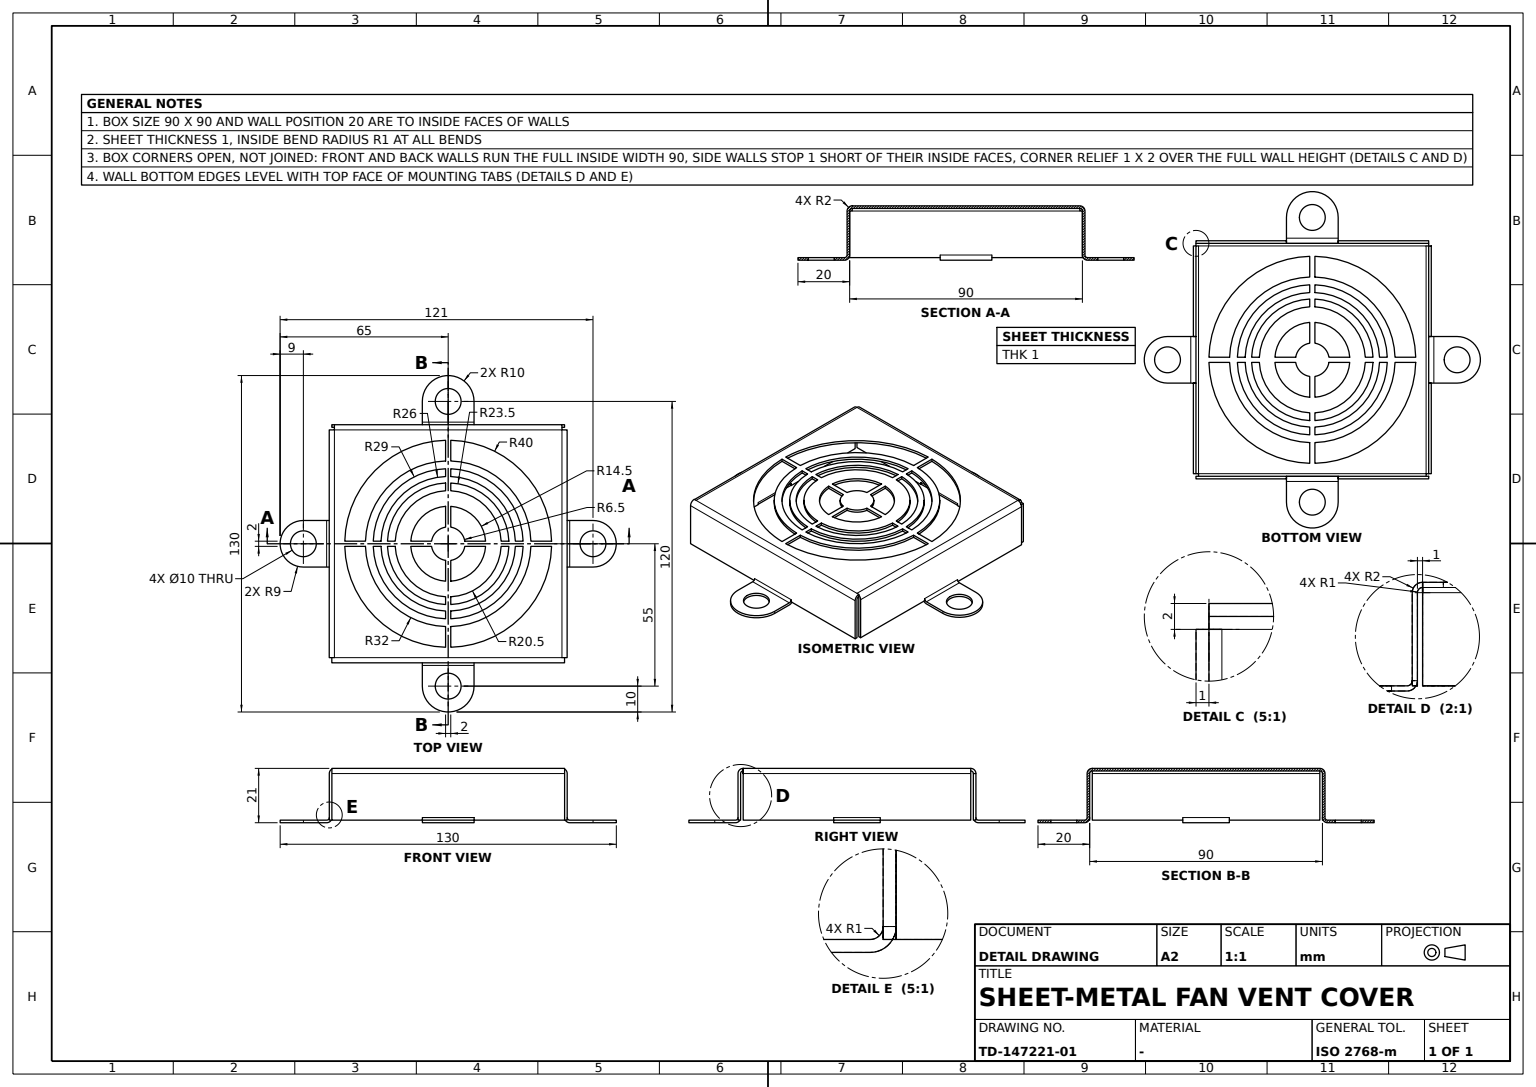
solid
v1 (14.465476,-1,0)
v2 (14.465476,-1,1)
e1 v1 v2 LINE
v3 (6.422616,-1,1)
e2 v2 v3 LINE
v4 (6.422616,-1,0)
e3 v4 v3 LINE
e4 v1 v4 LINE
face PLANE(AX(P(-10.444046,-1,1),D(0,1,0),D(1,0,0))) rev [e1 e2 -e3 -e4]
v5 (1,25.982753,1)
v6 (25.982753,1,1)
e5 v5 v6 CIRCLE(AX(P(0,0,1),D(0,0,1),D(1,0,0)),26.00199) rev
v7 (25.982753,1,0)
e6 v7 v6 LINE
v8 (1,25.982753,0)
e7 v8 v7 CIRCLE(AX(P(0,0,0),D(0,0,1),D(1,0,0)),26.00199) rev
e8 v8 v5 LINE
face CYL(AX(P(0,0,1),D(0,0,1),D(0,1,0)),26.00199) [e5 -e6 -e7 e8]
v9 (-56,9,-20)
v10 (-55.999997,9,-19)
e9 v9 v10 LINE
v11 (-47,9,-19)
e10 v10 v11 LINE
v12 (-46,9,-18)
e11 v11 v12 CIRCLE(AX(P(-47,9,-18),D(0,-1,0),D(0,0,-1)),1)
v13 (-45,9,-18)
e12 v13 v12 LINE
v14 (-47,9,-20)
e13 v14 v13 CIRCLE(AX(P(-47,9,-18),D(0,-1,0),D(0,0,-1)),2)
e14 v9 v14 LINE
face PLANE(AX(P(56,9,-20),D(0,-1,0),D(1,0,0))) rev [e9 e10 e11 -e12 -e13 -e14]
v15 (-61,0,-20)
e15 v15 v15 CIRCLE(AX(P(-56,0,-20),D(0,0,-1),D(-1,0,0)),5) rev
v16 (-61,0,-19)
e16 v16 v16 CIRCLE(AX(P(-56,0,-19),D(0,0,-1),D(-1,0,0)),5) rev
face CYL(AX(P(-56,0,-19),D(0,0,-1),D(0,1,0)),5) rev [-e15] [e16]
v17 (-1,-14.465476,0)
v18 (-14.465476,-1,0)
e17 v17 v18 CIRCLE(AX(P(0,0,0),D(0,0,1),D(1,0,0)),14.5) rev
v19 (-14.465476,-1,1)
e18 v18 v19 LINE
v20 (-1,-14.465476,1)
e19 v20 v19 CIRCLE(AX(P(0,0,1),D(0,0,1),D(1,0,0)),14.5) rev
e20 v17 v20 LINE
face CYL(AX(P(0,0,1),D(0,0,1),D(0,1,0)),14.5) rev [e17 e18 -e19 -e20]
v21 (-56,-9,-20)
e21 v21 v9 CIRCLE(AX(P(-56,0,-20),D(0,0,-1),D(-1,0,0)),9)
v22 (-56,-9,-19)
e22 v21 v22 LINE
e23 v22 v10 CIRCLE(AX(P(-56,0,-19),D(0,0,-1),D(-1,0,0)),9)
face CYL(AX(P(-56,0,-19),D(0,0,-1),D(0,1,0)),9) [-e9 -e21 e22 e23]
v23 (10,45,-18)
v24 (10,45,-19)
e24 v23 v24 LINE
v25 (10,46,-18)
e25 v23 v25 LINE
v26 (10,46,-19)
e26 v25 v26 LINE
e27 v24 v26 LINE
face PLANE(AX(P(10,-45,-18),D(-1,0,0),D(0,-0.382683432,-0.923879533))) [-e24 e25 e26 -e27]
v27 (-31.984371,-1,0)
v28 (-31.984371,-1,1)
e28 v27 v28 LINE
v29 (-1,-31.984371,0)
e29 v27 v29 CIRCLE(AX(P(0,0,0),D(0,0,1),D(1,0,0)),32)
v30 (-1,-31.984371,1)
e30 v29 v30 LINE
e31 v28 v30 CIRCLE(AX(P(0,0,1),D(0,0,1),D(1,0,0)),32)
face CYL(AX(P(0,0,1),D(0,0,1),D(0,1,0)),32) [-e28 e29 e30 -e31]
v31 (1,-14.465476,0)
e32 v1 v31 CIRCLE(AX(P(0,0,0),D(0,0,1),D(1,0,0)),14.5) rev
v32 (1,-14.465476,1)
e33 v31 v32 LINE
e34 v2 v32 CIRCLE(AX(P(0,0,1),D(0,0,1),D(1,0,0)),14.5) rev
face CYL(AX(P(0,0,1),D(0,0,1),D(0,1,0)),14.5) rev [e32 e33 -e34 -e1]
v33 (-45,46,-19)
v34 (-45,46,-1)
e35 v33 v34 LINE
v35 (-45,45,-19)
e36 v35 v33 LINE
v36 (-45,45,-1)
e37 v35 v36 LINE
e38 v36 v34 LINE
face PLANE(AX(P(-45,46,-10),D(-1,0,0),D(0,1,0))) [-e35 -e36 e37 e38]
v37 (1,14.465476,1)
v38 (14.465476,1,1)
e39 v37 v38 CIRCLE(AX(P(0,0,1),D(0,0,1),D(1,0,0)),14.5) rev
v39 (1,14.465476,0)
e40 v39 v37 LINE
v40 (14.465476,1,0)
e41 v39 v40 CIRCLE(AX(P(0,0,0),D(0,0,1),D(1,0,0)),14.5) rev
e42 v40 v38 LINE
face CYL(AX(P(0,0,1),D(0,0,1),D(0,1,0)),14.5) rev [-e39 -e40 e41 e42]
v41 (6.422616,1,0)
e43 v41 v40 LINE
v42 (6.422616,1,1)
e44 v41 v42 LINE
e45 v42 v38 LINE
face PLANE(AX(P(-10.444046,1,1),D(0,1,0),D(1,0,0))) [-e42 -e43 e44 e45]
v43 (-46,44,-19)
v44 (-46,9,-19)
e46 v43 v44 LINE
v45 (-45,44,-19)
e47 v43 v45 LINE
v46 (-45,9,-19)
e48 v45 v46 LINE
e49 v46 v44 LINE
face PLANE(AX(P(46,0,-19),D(0,0,-1),D(0,1,0))) [-e46 e47 e48 e49]
v47 (-1,14.465476,0)
v48 (-1,14.465476,1)
e50 v47 v48 LINE
v49 (-14.465476,1,1)
e51 v48 v49 CIRCLE(AX(P(0,0,1),D(0,0,1),D(1,0,0)),14.5)
v50 (-14.465476,1,0)
e52 v50 v49 LINE
e53 v47 v50 CIRCLE(AX(P(0,0,0),D(0,0,1),D(1,0,0)),14.5)
face CYL(AX(P(0,0,1),D(0,0,1),D(0,1,0)),14.5) rev [e50 e51 -e52 -e53]
v51 (45,45,-1)
v52 (45,46,-1)
e54 v51 v52 LINE
v53 (45,45,-19)
e55 v53 v51 LINE
v54 (45,46,-19)
e56 v53 v54 LINE
e57 v54 v52 LINE
face PLANE(AX(P(45,0,1),D(-1,0,0),D(0,1,0))) rev [-e54 -e55 e56 e57]
v55 (-45,-9,-18)
v56 (-46,-9,-18)
e58 v55 v56 LINE
v57 (-45,-9,-19)
e59 v55 v57 LINE
v58 (-46,-9,-19)
e60 v57 v58 LINE
e61 v56 v58 LINE
face PLANE(AX(P(56,-9,-20),D(0,-1,0),D(1,0,0))) rev [-e58 e59 e60 -e61]
e62 v12 v44 LINE
e63 v56 v12 LINE
v59 (-46,-44,-19)
e64 v58 v59 LINE
v60 (-46,-44,-1)
e65 v59 v60 LINE
v61 (-46,44,-1)
e66 v60 v61 LINE
e67 v61 v43 LINE
face PLANE(AX(P(-46,0,1),D(-1,0,0),D(0,1,0))) [e46 -e62 -e63 e61 e64 e65 e66 e67]
v62 (-1,25.982753,0)
v63 (-1,25.982753,1)
e68 v62 v63 LINE
v64 (-25.982753,1,0)
e69 v62 v64 CIRCLE(AX(P(0,0,0),D(0,0,1),D(1,0,0)),26.00199)
v65 (-25.982753,1,1)
e70 v64 v65 LINE
e71 v63 v65 CIRCLE(AX(P(0,0,1),D(0,0,1),D(1,0,0)),26.00199)
face CYL(AX(P(0,0,1),D(0,0,1),D(0,1,0)),26.00199) [-e68 e69 e70 -e71]
v66 (10,54.999996,-19)
v67 (10,47,-19)
e72 v66 v67 LINE
v68 (-10,55,-19)
e73 v68 v66 CIRCLE(AX(P(0,55,-19),D(0,0,-1),D(-1,0,0)),10)
v69 (-10,47,-19)
e74 v68 v69 LINE
e75 v67 v69 LINE
v70 (-5,55,-19)
e76 v70 v70 CIRCLE(AX(P(0,55,-19),D(0,0,-1),D(-1,0,0)),5) rev
face PLANE(AX(P(46,0,-19),D(0,0,-1),D(0,1,0))) rev [-e72 -e73 e74 -e75] [-e76]
e77 v54 v26 LINE
v71 (-10,46,-18)
e78 v25 v71 LINE
v72 (-10,46,-19)
e79 v71 v72 LINE
e80 v72 v33 LINE
v73 (-44,46,-1)
e81 v34 v73 LINE
v74 (44,46,-1)
e82 v74 v73 LINE
e83 v74 v52 LINE
face PLANE(AX(P(0,46,1),D(0,-1,0),D(-1,0,0))) rev [e77 -e26 e78 e79 e80 e35 e81 -e82 e83 -e57]
v75 (-6.422616,-1,0)
v76 (-6.422616,-1,1)
e84 v75 v76 LINE
v77 (-1,-6.422616,0)
e85 v77 v75 CIRCLE(AX(P(0,0,0),D(0,0,1),D(1,0,0)),6.5) rev
v78 (-1,-6.422616,1)
e86 v77 v78 LINE
e87 v78 v76 CIRCLE(AX(P(0,0,1),D(0,0,1),D(1,0,0)),6.5) rev
face CYL(AX(P(0,0,1),D(0,0,1),D(0,1,0)),6.5) [-e84 -e85 e86 e87]
v79 (1,28.982753,0)
v80 (1,28.982753,1)
e88 v79 v80 LINE
e89 v5 v80 LINE
e90 v8 v79 LINE
face PLANE(AX(P(1,-10.444046,1),D(1,0,0),D(0,1,0))) [e88 -e89 -e8 e90]
v81 (39.987498,-1,0)
v82 (39.987498,-1,1)
e91 v81 v82 LINE
v83 (31.984371,-1,1)
e92 v83 v82 LINE
v84 (31.984371,-1,0)
e93 v84 v83 LINE
e94 v84 v81 LINE
face PLANE(AX(P(-10.444046,-1,1),D(0,1,0),D(1,0,0))) rev [e91 -e92 -e93 e94]
v85 (47,-9,-20)
v86 (47,9,-20)
e95 v85 v86 LINE
v87 (56,9,-20)
e96 v87 v86 LINE
v88 (56,-9,-20)
e97 v87 v88 CIRCLE(AX(P(56,0,-20),D(0,0,-1),D(-1,0,0)),9)
e98 v85 v88 LINE
v89 (51,0,-20)
e99 v89 v89 CIRCLE(AX(P(56,0,-20),D(0,0,-1),D(-1,0,0)),5)
face PLANE(AX(P(46,0,-20),D(0,0,-1),D(0,1,0))) [e95 -e96 e97 -e98] [-e99]
v90 (47,-9,-19)
v91 (56,-9,-19)
e100 v90 v91 LINE
v92 (46,-9,-18)
e101 v92 v90 CIRCLE(AX(P(47,-9,-18),D(0,-1,0),D(0,0,-1)),1)
v93 (45,-9,-18)
e102 v93 v92 LINE
e103 v93 v85 CIRCLE(AX(P(47,-9,-18),D(0,-1,0),D(0,0,-1)),2)
e104 v88 v91 LINE
face PLANE(AX(P(56,-9,-20),D(0,-1,0),D(1,0,0))) [-e100 -e101 -e102 e103 e98 e104]
v94 (46,-44,-1)
v95 (44,-44,1)
e105 v94 v95 CIRCLE(AX(P(44,-44,-1),D(0,1,0),D(0,0,1)),2) rev
v96 (46,44,-1)
e106 v94 v96 LINE
v97 (44,44,1)
e107 v96 v97 CIRCLE(AX(P(44,44,-1),D(0,1,0),D(0,0,1)),2) rev
e108 v95 v97 LINE
face CYL(AX(P(44,-44,-1),D(0,1,0),D(0,0,1)),2) [-e105 e106 e107 -e108]
v98 (10,-45,-18)
v99 (10,-45,-19)
e109 v98 v99 LINE
v100 (10,-46,-19)
e110 v99 v100 LINE
v101 (10,-46,-18)
e111 v101 v100 LINE
e112 v98 v101 LINE
face PLANE(AX(P(10,-45,-18),D(-1,0,0),D(0,-0.382683432,-0.923879533))) [e109 e110 -e111 -e112]
v102 (-44,44,0)
v103 (-45,44,-1)
e113 v102 v103 CIRCLE(AX(P(-44,44,-1),D(0,1,0),D(0,0,1)),1) rev
v104 (-44,-44,0)
e114 v104 v102 LINE
v105 (-45,-44,-1)
e115 v104 v105 CIRCLE(AX(P(-44,-44,-1),D(0,1,0),D(0,0,1)),1) rev
e116 v105 v103 LINE
face CYL(AX(P(-44,44,-1),D(0,-1,0),D(0,0,1)),1) rev [-e113 -e114 e115 e116]
v106 (1,-39.987498,0)
v107 (1,-39.987498,1)
e117 v106 v107 LINE
v108 (1,-31.984371,0)
e118 v108 v106 LINE
v109 (1,-31.984371,1)
e119 v108 v109 LINE
e120 v109 v107 LINE
face PLANE(AX(P(1,-10.444046,1),D(1,0,0),D(0,1,0))) [-e117 -e118 e119 e120]
v110 (-28.982753,-1,0)
v111 (-28.982753,-1,1)
e121 v110 v111 LINE
v112 (-1,-28.982753,1)
e122 v112 v111 CIRCLE(AX(P(0,0,1),D(0,0,1),D(1,0,0)),29) rev
v113 (-1,-28.982753,0)
e123 v113 v112 LINE
e124 v113 v110 CIRCLE(AX(P(0,0,0),D(0,0,1),D(1,0,0)),29) rev
face CYL(AX(P(0,0,1),D(0,0,1),D(0,1,0)),29) rev [e121 -e122 -e123 e124]
v114 (45,44,-1)
v115 (44,44,0)
e125 v114 v115 CIRCLE(AX(P(44,44,-1),D(0,1,0),D(0,0,1)),1) rev
v116 (45,-44,-1)
e126 v116 v114 LINE
v117 (44,-44,0)
e127 v116 v117 CIRCLE(AX(P(44,-44,-1),D(0,1,0),D(0,0,1)),1) rev
e128 v117 v115 LINE
face CYL(AX(P(44,-44,-1),D(0,1,0),D(0,0,1)),1) rev [-e125 -e126 e127 e128]
v118 (-31.984371,1,0)
v119 (-39.987498,1,0)
e129 v118 v119 LINE
v120 (-39.987498,1,1)
e130 v119 v120 LINE
v121 (-31.984371,1,1)
e131 v121 v120 LINE
e132 v118 v121 LINE
face PLANE(AX(P(-10.444046,1,1),D(0,1,0),D(1,0,0))) [e129 e130 -e131 -e132]
v122 (39.987498,1,0)
v123 (31.984371,1,0)
e133 v122 v123 LINE
v124 (31.984371,1,1)
e134 v123 v124 LINE
v125 (39.987498,1,1)
e135 v125 v124 LINE
e136 v122 v125 LINE
face PLANE(AX(P(-10.444046,1,1),D(0,1,0),D(1,0,0))) [e133 e134 -e135 -e136]
v126 (25.982753,-1,0)
v127 (25.982753,-1,1)
e137 v126 v127 LINE
v128 (28.982753,-1,0)
e138 v126 v128 LINE
v129 (28.982753,-1,1)
e139 v128 v129 LINE
e140 v127 v129 LINE
face PLANE(AX(P(-10.444046,-1,1),D(0,1,0),D(1,0,0))) rev [-e137 e138 e139 -e140]
v130 (10,47,-20)
e141 v23 v130 CIRCLE(AX(P(10,47,-18),D(-1,0,0),D(0,0,1)),2) rev
v131 (-10,45,-18)
e142 v23 v131 LINE
v132 (-10,47,-20)
e143 v131 v132 CIRCLE(AX(P(-10,47,-18),D(-1,0,0),D(0,0,1)),2) rev
e144 v130 v132 LINE
face CYL(AX(P(-10,47,-18),D(1,0,0),D(0,-1,0)),2) [-e141 e142 e143 -e144]
v133 (1,-6.422616,0)
e145 v31 v133 LINE
v134 (1,-6.422616,1)
e146 v133 v134 LINE
e147 v32 v134 LINE
face PLANE(AX(P(1,-10.444046,1),D(1,0,0),D(0,1,0))) [-e33 e145 e146 -e147]
v135 (1,-25.982753,0)
e148 v135 v126 CIRCLE(AX(P(0,0,0),D(0,0,1),D(1,0,0)),26.00199)
v136 (1,-25.982753,1)
e149 v136 v127 CIRCLE(AX(P(0,0,1),D(0,0,1),D(1,0,0)),26.00199)
e150 v135 v136 LINE
face CYL(AX(P(0,0,1),D(0,0,1),D(0,1,0)),26.00199) [e148 e137 -e149 -e150]
v137 (45,-45,-1)
v138 (-45,-45,-1)
e151 v137 v138 LINE
v139 (-45,-44,0)
e152 v139 v138 CIRCLE(AX(P(-45,-44,-1),D(-1,0,0),D(0,0,1)),1) rev
e153 v139 v104 LINE
e154 v117 v104 LINE
v140 (45,-44,0)
e155 v140 v117 LINE
e156 v140 v137 CIRCLE(AX(P(45,-44,-1),D(-1,0,0),D(0,0,1)),1) rev
face CYL(AX(P(-45,-44,-1),D(1,0,0),D(0,0,1)),1) rev [e151 -e152 e153 -e154 -e155 e156]
v141 (46,-9,-19)
e157 v92 v141 LINE
v142 (45,-9,-19)
e158 v142 v141 LINE
e159 v93 v142 LINE
face PLANE(AX(P(56,-9,-20),D(0,-1,0),D(1,0,0))) rev [e157 -e158 -e159 e102]
v143 (-28.982753,1,1)
e160 v65 v143 LINE
v144 (-28.982753,1,0)
e161 v64 v144 LINE
e162 v144 v143 LINE
face PLANE(AX(P(-10.444046,1,1),D(0,1,0),D(1,0,0))) [-e160 -e70 e161 e162]
v145 (-44,44,1)
e163 v102 v145 LINE
e164 v145 v73 CIRCLE(AX(P(-44,44,-1),D(-1,0,0),D(0,0,1)),2)
v146 (-44,45,-1)
e165 v146 v73 LINE
e166 v102 v146 CIRCLE(AX(P(-44,44,-1),D(-1,0,0),D(0,0,1)),1)
face PLANE(AX(P(-44,44,0),D(-1,0,0),D(0,0.923879533,-0.382683432))) [e163 e164 -e165 -e166]
v147 (44,45,-1)
e167 v147 v51 LINE
e168 v147 v146 LINE
e169 v36 v146 LINE
v148 (-10,45,-19)
e170 v35 v148 LINE
e171 v131 v148 LINE
e172 v24 v53 LINE
face PLANE(AX(P(0,45,1),D(0,-1,0),D(-1,0,0))) [-e167 e168 -e169 -e37 e170 -e171 -e142 e24 e172 e55]
v149 (45,-44,1)
e173 v149 v95 LINE
e174 v140 v149 LINE
e175 v117 v95 LINE
face PLANE(AX(P(46,-44,-10),D(0,1,0),D(1,0,0))) [-e173 -e174 e155 e175]
v150 (-5,-55,-20)
e176 v150 v150 CIRCLE(AX(P(0,-55,-20),D(0,0,-1),D(-1,0,0)),5) rev
v151 (-5,-55,-19)
e177 v151 v151 CIRCLE(AX(P(0,-55,-19),D(0,0,-1),D(-1,0,0)),5) rev
face CYL(AX(P(0,-55,-19),D(0,0,-1),D(-1,0,0)),5) rev [-e176] [e177]
v152 (45,44,-19)
e178 v152 v114 LINE
v153 (45,9,-19)
e179 v152 v153 LINE
v154 (45,9,-18)
e180 v154 v153 LINE
e181 v93 v154 LINE
v155 (45,-44,-19)
e182 v142 v155 LINE
e183 v116 v155 LINE
face PLANE(AX(P(45,0,1),D(-1,0,0),D(0,1,0))) [-e178 e179 -e180 -e181 e159 e182 -e183 e126]
v156 (23.478714,1,0)
v157 (1,23.478714,0)
e184 v156 v157 CIRCLE(AX(P(0,0,0),D(0,0,1),D(1,0,0)),23.5)
v158 (23.478714,1,1)
e185 v156 v158 LINE
v159 (1,23.478714,1)
e186 v158 v159 CIRCLE(AX(P(0,0,1),D(0,0,1),D(1,0,0)),23.5)
e187 v157 v159 LINE
face CYL(AX(P(0,0,1),D(0,0,1),D(0,1,0)),23.5) rev [-e184 e185 e186 -e187]
v160 (10,-47,-20)
e188 v160 v98 CIRCLE(AX(P(10,-47,-18),D(-1,0,0),D(0,0,1)),2) rev
v161 (10,-47,-19)
e189 v161 v101 CIRCLE(AX(P(10,-47,-18),D(-1,0,0),D(0,0,1)),1) rev
v162 (10,-55,-19)
e190 v162 v161 LINE
v163 (10,-54.999996,-20)
e191 v163 v162 LINE
e192 v163 v160 LINE
face PLANE(AX(P(10,-45,-18),D(-1,0,0),D(0,-0.382683432,-0.923879533))) rev [e188 e112 -e189 -e190 -e191 e192]
e193 v109 v83 CIRCLE(AX(P(0,0,1),D(0,0,1),D(1,0,0)),32)
e194 v108 v84 CIRCLE(AX(P(0,0,0),D(0,0,1),D(1,0,0)),32)
face CYL(AX(P(0,0,1),D(0,0,1),D(0,1,0)),32) [-e193 -e119 e194 e93]
v164 (-10,-55,-19)
v165 (-10,-47,-19)
e195 v164 v165 LINE
e196 v162 v164 CIRCLE(AX(P(0,-55,-19),D(0,0,-1),D(-1,0,0)),10)
e197 v161 v165 LINE
face PLANE(AX(P(46,0,-19),D(0,0,-1),D(0,1,0))) rev [-e195 -e196 e190 e197] [-e177]
v166 (-45,-44,1)
v167 (-44,-44,1)
e198 v166 v167 LINE
e199 v104 v167 LINE
e200 v139 v166 LINE
face PLANE(AX(P(46,-44,-10),D(0,1,0),D(1,0,0))) [e198 -e199 -e153 e200]
v168 (-10,-55,-20)
e201 v163 v168 CIRCLE(AX(P(0,-55,-20),D(0,0,-1),D(-1,0,0)),10)
v169 (-10,-47,-20)
e202 v168 v169 LINE
e203 v160 v169 LINE
face PLANE(AX(P(46,0,-20),D(0,0,-1),D(0,1,0))) [e201 e202 -e203 -e192] [e176]
e204 v131 v71 LINE
e205 v148 v72 LINE
face PLANE(AX(P(-10,-45,-18),D(-1,0,0),D(0,-0.382683432,-0.923879533))) rev [-e204 e171 e205 -e79]
v170 (20.478714,1,1)
e206 v158 v170 LINE
v171 (20.478714,1,0)
e207 v156 v171 LINE
e208 v171 v170 LINE
face PLANE(AX(P(-10.444046,1,1),D(0,1,0),D(1,0,0))) [-e206 -e185 e207 e208]
v172 (46,9,-19)
e209 v153 v172 LINE
v173 (46,9,-18)
e210 v173 v172 LINE
e211 v154 v173 LINE
face PLANE(AX(P(56,9,-20),D(0,-1,0),D(1,0,0))) [e180 e209 -e210 -e211]
v174 (-1,-25.982753,0)
e212 v174 v113 LINE
v175 (-1,-25.982753,1)
e213 v175 v112 LINE
e214 v174 v175 LINE
face PLANE(AX(P(-1,10.444046,1),D(1,0,0),D(0,1,0))) rev [e212 e123 -e213 -e214]
v176 (-1,-39.987498,0)
v177 (-1,-39.987498,1)
e215 v176 v177 LINE
e216 v30 v177 LINE
e217 v29 v176 LINE
face PLANE(AX(P(-1,10.444046,1),D(1,0,0),D(0,1,0))) rev [e215 -e216 -e30 e217]
e218 v77 v17 LINE
e219 v78 v20 LINE
face PLANE(AX(P(-1,10.444046,1),D(1,0,0),D(0,1,0))) rev [-e86 e218 e20 -e219]
e220 v97 v74 CIRCLE(AX(P(44,44,-1),D(-1,0,0),D(0,0,1)),2)
e221 v115 v97 LINE
e222 v115 v147 CIRCLE(AX(P(44,44,-1),D(-1,0,0),D(0,0,1)),1)
e223 v147 v74 LINE
face PLANE(AX(P(44,44,0),D(-1,0,0),D(0,0.923879533,-0.382683432))) rev [-e220 -e221 e222 e223]
v178 (-10,-46,-18)
e224 v101 v178 LINE
e225 v165 v178 CIRCLE(AX(P(-10,-47,-18),D(-1,0,0),D(0,0,1)),1) rev
face CYL(AX(P(10,-47,-18),D(-1,0,0),D(0,1,0)),1) rev [e224 -e225 -e197 e189]
v179 (-1,6.422616,0)
v180 (-1,6.422616,1)
e226 v179 v180 LINE
v181 (-6.422616,1,0)
e227 v179 v181 CIRCLE(AX(P(0,0,0),D(0,0,1),D(1,0,0)),6.5)
v182 (-6.422616,1,1)
e228 v181 v182 LINE
e229 v180 v182 CIRCLE(AX(P(0,0,1),D(0,0,1),D(1,0,0)),6.5)
face CYL(AX(P(0,0,1),D(0,0,1),D(0,1,0)),6.5) [-e226 e227 e228 -e229]
v183 (-47,-9,-19)
e230 v183 v56 CIRCLE(AX(P(-47,-9,-18),D(0,-1,0),D(0,0,-1)),1)
e231 v22 v183 LINE
v184 (-47,-9,-20)
e232 v21 v184 LINE
e233 v184 v55 CIRCLE(AX(P(-47,-9,-18),D(0,-1,0),D(0,0,-1)),2)
face PLANE(AX(P(56,-9,-20),D(0,-1,0),D(1,0,0))) [e58 -e230 -e231 -e22 e232 e233]
v185 (28.982753,1,1)
e234 v185 v6 LINE
v186 (28.982753,1,0)
e235 v186 v185 LINE
e236 v186 v7 LINE
face PLANE(AX(P(-10.444046,1,1),D(0,1,0),D(1,0,0))) [e6 -e234 -e235 e236]
face PLANE(AX(P(46,0,-19),D(0,0,-1),D(0,1,0))) [-e77 -e56 -e172 e27]
v187 (1,6.422616,0)
e237 v187 v39 LINE
v188 (1,6.422616,1)
e238 v188 v37 LINE
e239 v187 v188 LINE
face PLANE(AX(P(1,-10.444046,1),D(1,0,0),D(0,1,0))) [e237 e40 -e238 -e239]
face PLANE(AX(P(44.5,46,-1),D(0,0,-1),D(1,0,0))) rev [e165 -e81 -e38 e169]
v189 (1,-28.982753,1)
e240 v136 v189 LINE
v190 (1,-28.982753,0)
e241 v190 v189 LINE
e242 v135 v190 LINE
face PLANE(AX(P(1,-10.444046,1),D(1,0,0),D(0,1,0))) [e240 -e241 -e242 e150]
v191 (-1,23.478714,0)
v192 (-1,20.478714,0)
e243 v191 v192 LINE
v193 (-1,20.478714,1)
e244 v192 v193 LINE
v194 (-1,23.478714,1)
e245 v194 v193 LINE
e246 v191 v194 LINE
face PLANE(AX(P(-1,10.444046,1),D(1,0,0),D(0,1,0))) rev [e243 e244 -e245 -e246]
v195 (51,0,-19)
e247 v195 v195 CIRCLE(AX(P(56,0,-19),D(0,0,-1),D(-1,0,0)),5)
v196 (47,9,-19)
e248 v90 v196 LINE
v197 (56,9,-19)
e249 v197 v91 CIRCLE(AX(P(56,0,-19),D(0,0,-1),D(-1,0,0)),9)
e250 v197 v196 LINE
face PLANE(AX(P(46,0,-19),D(0,0,-1),D(0,1,0))) rev [e247] [-e248 e100 -e249 e250]
v198 (1,-20.478714,0)
v199 (1,-20.478714,1)
e251 v198 v199 LINE
v200 (1,-23.478714,1)
e252 v199 v200 LINE
v201 (1,-23.478714,0)
e253 v201 v200 LINE
e254 v198 v201 LINE
face PLANE(AX(P(1,-10.444046,1),D(1,0,0),D(0,1,0))) [e251 e252 -e253 -e254]
v202 (-25.982753,-1,0)
e255 v202 v174 CIRCLE(AX(P(0,0,0),D(0,0,1),D(1,0,0)),26.00199)
v203 (-25.982753,-1,1)
e256 v203 v175 CIRCLE(AX(P(0,0,1),D(0,0,1),D(1,0,0)),26.00199)
e257 v202 v203 LINE
face CYL(AX(P(0,0,1),D(0,0,1),D(0,1,0)),26.00199) [e255 e214 -e256 -e257]
e258 v183 v11 LINE
face PLANE(AX(P(46,0,-19),D(0,0,-1),D(0,1,0))) rev [e258 -e10 -e23 e231] [-e16]
e259 v167 v60 CIRCLE(AX(P(-44,-44,-1),D(0,1,0),D(0,0,1)),2) rev
v204 (-45,-44,-19)
e260 v59 v204 LINE
e261 v204 v105 LINE
face PLANE(AX(P(46,-44,-10),D(0,1,0),D(1,0,0))) rev [e199 e259 -e65 e260 e261 -e115]
e262 v87 v197 LINE
face CYL(AX(P(56,0,-19),D(0,0,-1),D(0,1,0)),9) [-e97 e262 e249 -e104]
v205 (45,-46,-1)
e263 v149 v205 CIRCLE(AX(P(45,-44,-1),D(-1,0,0),D(0,0,1)),2) rev
v206 (45,-46,-19)
e264 v206 v205 LINE
v207 (45,-45,-19)
e265 v206 v207 LINE
e266 v207 v137 LINE
face PLANE(AX(P(45,0,1),D(-1,0,0),D(0,1,0))) rev [e263 -e264 e265 e266 -e156 e174]
e267 v99 v207 LINE
e268 v100 v206 LINE
face PLANE(AX(P(46,0,-19),D(0,0,-1),D(0,1,0))) [-e110 e267 -e265 -e268]
v208 (23.478714,-1,0)
e269 v208 v201 CIRCLE(AX(P(0,0,0),D(0,0,1),D(1,0,0)),23.5) rev
v209 (23.478714,-1,1)
e270 v209 v200 CIRCLE(AX(P(0,0,1),D(0,0,1),D(1,0,0)),23.5) rev
e271 v208 v209 LINE
face CYL(AX(P(0,0,1),D(0,0,1),D(0,1,0)),23.5) rev [e269 e253 -e270 -e271]
v210 (-5,55,-20)
e272 v210 v210 CIRCLE(AX(P(0,55,-20),D(0,0,-1),D(-1,0,0)),5) rev
face CYL(AX(P(0,55,-19),D(0,0,-1),D(-1,0,0)),5) rev [-e272] [e76]
e273 v145 v61 CIRCLE(AX(P(-44,44,-1),D(0,1,0),D(0,0,1)),2) rev
e274 v103 v45 LINE
face PLANE(AX(P(46,44,-10),D(0,1,0),D(1,0,0))) [-e273 -e163 e113 e274 -e47 -e67]
e275 v92 v173 LINE
e276 v173 v196 CIRCLE(AX(P(47,9,-18),D(0,-1,0),D(0,0,-1)),1)
face CYL(AX(P(47,9,-18),D(0,-1,0),D(-1,0,0)),1) rev [-e275 e101 e248 -e276]
v211 (-39.987498,-1,1)
e277 v28 v211 LINE
v212 (-39.987498,-1,0)
e278 v212 v211 LINE
e279 v27 v212 LINE
face PLANE(AX(P(-10.444046,-1,1),D(0,1,0),D(1,0,0))) rev [e28 e277 -e278 -e279]
v213 (46,-44,-19)
e280 v94 v213 LINE
e281 v213 v141 LINE
v214 (46,44,-19)
e282 v172 v214 LINE
e283 v214 v96 LINE
face PLANE(AX(P(46,0,1),D(-1,0,0),D(0,1,0))) rev [e280 e281 -e157 e275 e210 e282 e283 -e106]
e284 v177 v211 CIRCLE(AX(P(0,0,1),D(0,0,1),D(1,0,0)),40) rev
e285 v176 v212 CIRCLE(AX(P(0,0,0),D(0,0,1),D(1,0,0)),40) rev
face CYL(AX(P(0,0,1),D(0,0,1),D(0,1,0)),40) rev [-e284 -e215 e285 e278]
e286 v25 v67 CIRCLE(AX(P(10,47,-18),D(-1,0,0),D(0,0,1)),1) rev
e287 v71 v69 CIRCLE(AX(P(-10,47,-18),D(-1,0,0),D(0,0,1)),1) rev
face CYL(AX(P(-10,47,-18),D(1,0,0),D(0,-1,0)),1) rev [e286 e75 -e287 -e78]
v215 (-45,-46,-19)
v216 (-10,-46,-19)
e288 v215 v216 LINE
v217 (-45,-45,-19)
e289 v215 v217 LINE
v218 (-10,-45,-19)
e290 v217 v218 LINE
e291 v218 v216 LINE
face PLANE(AX(P(46,0,-19),D(0,0,-1),D(0,1,0))) [-e288 e289 e290 e291]
face PLANE(AX(P(46,0,-19),D(0,0,-1),D(0,1,0))) [e36 -e80 -e205 -e170]
e292 v203 v111 LINE
e293 v202 v110 LINE
face PLANE(AX(P(-10.444046,-1,1),D(0,1,0),D(1,0,0))) rev [e292 -e121 -e293 e257]
v219 (20.478714,-1,0)
e294 v198 v219 CIRCLE(AX(P(0,0,0),D(0,0,1),D(1,0,0)),20.503115)
v220 (20.478714,-1,1)
e295 v219 v220 LINE
e296 v199 v220 CIRCLE(AX(P(0,0,1),D(0,0,1),D(1,0,0)),20.503115)
face CYL(AX(P(0,0,1),D(0,0,1),D(0,1,0)),20.503115) [-e251 e294 e295 -e296]
face PLANE(AX(P(44.5,46,-1),D(0,0,-1),D(1,0,0))) rev [e54 -e83 -e223 e167]
v221 (-1,39.987498,0)
e297 v119 v221 CIRCLE(AX(P(0,0,0),D(0,0,1),D(1,0,0)),40) rev
v222 (-1,39.987498,1)
e298 v221 v222 LINE
e299 v120 v222 CIRCLE(AX(P(0,0,1),D(0,0,1),D(1,0,0)),40) rev
face CYL(AX(P(0,0,1),D(0,0,1),D(0,1,0)),40) rev [-e130 e297 e298 -e299]
e300 v184 v14 LINE
face PLANE(AX(P(46,0,-20),D(0,0,-1),D(0,1,0))) [-e300 -e232 e21 e14] [e15]
e301 v3 v134 CIRCLE(AX(P(0,0,1),D(0,0,1),D(1,0,0)),6.5) rev
e302 v4 v133 CIRCLE(AX(P(0,0,0),D(0,0,1),D(1,0,0)),6.5) rev
face CYL(AX(P(0,0,1),D(0,0,1),D(0,1,0)),6.5) [e301 -e146 -e302 e3]
e303 v167 v145 LINE
face CYL(AX(P(-44,44,-1),D(0,-1,0),D(0,0,1)),2) [-e66 -e259 e303 e273]
v223 (-45,-46,-1)
e304 v205 v223 LINE
e305 v215 v223 LINE
e306 v178 v216 LINE
face PLANE(AX(P(0,-46,1),D(0,-1,0),D(-1,0,0))) [e264 e304 -e305 e288 -e306 -e224 e111 e268]
v224 (1,39.987498,0)
v225 (1,39.987498,1)
e307 v224 v225 LINE
v226 (1,31.984371,1)
e308 v226 v225 LINE
v227 (1,31.984371,0)
e309 v227 v226 LINE
e310 v227 v224 LINE
face PLANE(AX(P(1,-10.444046,1),D(1,0,0),D(0,1,0))) [e307 -e308 -e309 e310]
v228 (1,20.478714,1)
e311 v170 v228 CIRCLE(AX(P(0,0,1),D(0,0,1),D(1,0,0)),20.503115)
v229 (1,20.478714,0)
e312 v171 v229 CIRCLE(AX(P(0,0,0),D(0,0,1),D(1,0,0)),20.503115)
e313 v229 v228 LINE
face CYL(AX(P(0,0,1),D(0,0,1),D(0,1,0)),20.503115) [-e311 -e208 e312 e313]
face CYL(AX(P(56,0,-19),D(0,0,-1),D(0,1,0)),5) rev [-e247] [e99]
e314 v154 v86 CIRCLE(AX(P(47,9,-18),D(0,-1,0),D(0,0,-1)),2)
face PLANE(AX(P(56,9,-20),D(0,-1,0),D(1,0,0))) rev [-e314 e211 e276 -e250 -e262 e96]
e315 v168 v164 LINE
face CYL(AX(P(0,-55,-19),D(0,0,-1),D(-1,0,0)),10) [-e201 e191 e196 -e315]
v230 (-1,-20.478714,1)
v231 (-1,-23.478714,1)
e316 v230 v231 LINE
v232 (-1,-20.478714,0)
e317 v232 v230 LINE
v233 (-1,-23.478714,0)
e318 v232 v233 LINE
e319 v233 v231 LINE
face PLANE(AX(P(-1,10.444046,1),D(1,0,0),D(0,1,0))) rev [-e316 -e317 e318 e319]
v234 (-10,54.999996,-20)
e320 v234 v68 LINE
v235 (10,55,-20)
e321 v235 v66 LINE
e322 v234 v235 CIRCLE(AX(P(0,55,-20),D(0,0,-1),D(-1,0,0)),10)
face CYL(AX(P(0,55,-19),D(0,0,-1),D(-1,0,0)),10) [e320 e73 -e321 -e322]
e323 v217 v138 LINE
e324 v166 v223 CIRCLE(AX(P(-45,-44,-1),D(-1,0,0),D(0,0,1)),2) rev
face PLANE(AX(P(-45,46,-10),D(-1,0,0),D(0,1,0))) [-e200 e152 -e323 -e289 e305 -e324]
e325 v76 v19 LINE
e326 v75 v18 LINE
face PLANE(AX(P(-10.444046,-1,1),D(0,1,0),D(1,0,0))) rev [e325 -e18 -e326 e84]
e327 v115 v102 LINE
e328 v122 v224 CIRCLE(AX(P(0,0,0),D(0,0,1),D(1,0,0)),40)
e329 v123 v227 CIRCLE(AX(P(0,0,0),D(0,0,1),D(1,0,0)),32)
e330 v128 v190 CIRCLE(AX(P(0,0,0),D(0,0,1),D(1,0,0)),29) rev
e331 v219 v208 LINE
v236 (-20.478714,-1,0)
v237 (-23.478714,-1,0)
e332 v236 v237 LINE
e333 v233 v237 CIRCLE(AX(P(0,0,0),D(0,0,1),D(1,0,0)),23.5) rev
e334 v236 v232 CIRCLE(AX(P(0,0,0),D(0,0,1),D(1,0,0)),20.503115)
e335 v47 v179 LINE
e336 v181 v50 LINE
e337 v81 v106 CIRCLE(AX(P(0,0,0),D(0,0,1),D(1,0,0)),40) rev
v238 (-1,28.982753,0)
e338 v62 v238 LINE
e339 v144 v238 CIRCLE(AX(P(0,0,0),D(0,0,1),D(1,0,0)),29) rev
e340 v229 v157 LINE
v239 (-1,31.984371,0)
e341 v239 v118 CIRCLE(AX(P(0,0,0),D(0,0,1),D(1,0,0)),32)
e342 v239 v221 LINE
v240 (-23.478714,1,0)
e343 v191 v240 CIRCLE(AX(P(0,0,0),D(0,0,1),D(1,0,0)),23.5)
v241 (-20.478714,1,0)
e344 v241 v240 LINE
e345 v192 v241 CIRCLE(AX(P(0,0,0),D(0,0,1),D(1,0,0)),20.503115)
e346 v79 v186 CIRCLE(AX(P(0,0,0),D(0,0,1),D(1,0,0)),29) rev
e347 v41 v187 CIRCLE(AX(P(0,0,0),D(0,0,1),D(1,0,0)),6.5)
face PLANE(AX(P(0,0,0),D(0,0,1),D(0,1,0))) rev [-e128 e154 e114 -e327] [e328 -e310 -e329 -e133] [-e285 -e217 -e29 e279] [e242 -e330 -e138 -e148] [e254 -e269 -e331 -e294] [e332 -e333 -e318 -e334] [-e32 e4 e302 -e145] [-e17 -e218 e85 e326] [-e335 e53 -e336 -e227] [-e94 -e194 e118 -e337] [-e255 e293 -e124 -e212] [e338 -e339 -e161 -e69] [-e312 -e207 e184 -e340] [-e341 e342 -e297 -e129] [e343 -e344 -e345 -e243] [-e346 -e90 e7 -e236] [-e237 -e347 e43 -e41]
e348 v55 v13 LINE
face CYL(AX(P(-47,-9,-18),D(0,1,0),D(1,0,0)),2) [e300 e13 -e348 -e233]
e349 v82 v107 CIRCLE(AX(P(0,0,1),D(0,0,1),D(1,0,0)),40) rev
face CYL(AX(P(0,0,1),D(0,0,1),D(0,1,0)),40) rev [-e349 -e91 e337 e117]
e350 v129 v189 CIRCLE(AX(P(0,0,1),D(0,0,1),D(1,0,0)),29) rev
face CYL(AX(P(0,0,1),D(0,0,1),D(0,1,0)),29) rev [-e350 -e139 e330 e241]
e351 v182 v49 LINE
face PLANE(AX(P(-10.444046,1,1),D(0,1,0),D(1,0,0))) [e52 -e351 -e228 e336]
e352 v235 v130 LINE
face PLANE(AX(P(10,-45,-18),D(-1,0,0),D(0,-0.382683432,-0.923879533))) rev [-e286 -e25 e141 -e352 e321 e72]
v242 (-20.478714,-1,1)
v243 (-23.478714,-1,1)
e353 v242 v243 LINE
e354 v237 v243 LINE
e355 v236 v242 LINE
face PLANE(AX(P(-10.444046,-1,1),D(0,1,0),D(1,0,0))) rev [e353 -e354 -e332 e355]
e356 v231 v243 CIRCLE(AX(P(0,0,1),D(0,0,1),D(1,0,0)),23.5) rev
face CYL(AX(P(0,0,1),D(0,0,1),D(0,1,0)),23.5) rev [e354 -e356 -e319 e333]
e357 v125 v225 CIRCLE(AX(P(0,0,1),D(0,0,1),D(1,0,0)),40)
face CYL(AX(P(0,0,1),D(0,0,1),D(0,1,0)),40) rev [e136 e357 -e307 -e328]
e358 v124 v226 CIRCLE(AX(P(0,0,1),D(0,0,1),D(1,0,0)),32)
face CYL(AX(P(0,0,1),D(0,0,1),D(0,1,0)),32) [-e358 -e134 e329 e309]
v244 (-10,-45,-18)
e359 v244 v178 LINE
e360 v169 v244 CIRCLE(AX(P(-10,-47,-18),D(-1,0,0),D(0,0,1)),2) rev
face PLANE(AX(P(-10,-45,-18),D(-1,0,0),D(0,-0.382683432,-0.923879533))) [e315 e195 e225 -e359 -e360 -e202]
v245 (-23.478714,1,1)
e361 v194 v245 CIRCLE(AX(P(0,0,1),D(0,0,1),D(1,0,0)),23.5)
e362 v240 v245 LINE
face CYL(AX(P(0,0,1),D(0,0,1),D(0,1,0)),23.5) rev [e361 -e362 -e343 e246]
e363 v228 v159 LINE
face PLANE(AX(P(1,-10.444046,1),D(1,0,0),D(0,1,0))) [e340 e187 -e363 -e313]
face CYL(AX(P(47,9,-18),D(0,-1,0),D(-1,0,0)),2) [-e95 -e103 e181 e314]
e364 v57 v204 LINE
e365 v13 v46 LINE
face PLANE(AX(P(-45,46,-10),D(-1,0,0),D(0,1,0))) rev [-e48 -e274 -e116 -e261 -e364 -e59 e348 e365]
v246 (-20.478714,1,1)
e366 v241 v246 LINE
e367 v193 v246 CIRCLE(AX(P(0,0,1),D(0,0,1),D(1,0,0)),20.503115)
face CYL(AX(P(0,0,1),D(0,0,1),D(0,1,0)),20.503115) [-e244 e345 e366 -e367]
e368 v220 v209 LINE
face PLANE(AX(P(-10.444046,-1,1),D(0,1,0),D(1,0,0))) rev [-e295 e331 e271 -e368]
face PLANE(AX(P(56,9,-20),D(0,-1,0),D(1,0,0))) [e62 -e49 -e365 e12]
face PLANE(AX(P(46,0,-19),D(0,0,-1),D(0,1,0))) [-e64 -e60 e364 -e260]
e369 v234 v132 LINE
face PLANE(AX(P(-10,-45,-18),D(-1,0,0),D(0,-0.382683432,-0.923879533))) [-e74 -e320 e369 -e143 e204 e287]
e370 v244 v218 LINE
face PLANE(AX(P(-10,-45,-18),D(-1,0,0),D(0,-0.382683432,-0.923879533))) rev [-e291 -e370 e359 e306]
e371 v155 v213 LINE
face PLANE(AX(P(46,0,-19),D(0,0,-1),D(0,1,0))) [-e371 -e182 e158 -e281]
e372 v98 v244 LINE
face CYL(AX(P(10,-47,-18),D(-1,0,0),D(0,1,0)),2) [-e188 e203 e360 -e372]
face PLANE(AX(P(46,-44,-10),D(0,1,0),D(1,0,0))) rev [e371 -e280 e105 -e175 -e127 e183]
face PLANE(AX(P(46,0,-20),D(0,0,-1),D(0,1,0))) [e272] [-e369 e322 e352 e144]
e373 v97 v145 LINE
face CYL(AX(P(44,44,-1),D(-1,0,0),D(0,0,1)),2) [-e373 e220 e82 -e164]
v247 (-1,28.982753,1)
e374 v63 v247 LINE
e375 v238 v247 LINE
face PLANE(AX(P(-1,10.444046,1),D(1,0,0),D(0,1,0))) rev [-e338 e68 e374 -e375]
face CYL(AX(P(44,44,-1),D(-1,0,0),D(0,0,1)),1) rev [-e222 e327 e166 -e168]
e376 v48 v180 LINE
e377 v95 v167 LINE
v248 (-1,31.984371,1)
e378 v248 v222 LINE
e379 v248 v121 CIRCLE(AX(P(0,0,1),D(0,0,1),D(1,0,0)),32)
e380 v143 v247 CIRCLE(AX(P(0,0,1),D(0,0,1),D(1,0,0)),29) rev
e381 v246 v245 LINE
e382 v42 v188 CIRCLE(AX(P(0,0,1),D(0,0,1),D(1,0,0)),6.5)
e383 v80 v185 CIRCLE(AX(P(0,0,1),D(0,0,1),D(1,0,0)),29) rev
e384 v242 v230 CIRCLE(AX(P(0,0,1),D(0,0,1),D(1,0,0)),20.503115)
face PLANE(AX(P(0,0,1),D(0,0,1),D(0,1,0))) [e376 e229 e351 -e51] [e373 -e303 -e377 e108] [e299 -e378 e379 e131] [-e301 -e2 e34 e147] [e160 e380 -e374 e71] [-e186 e206 e311 e363] [-e361 e245 e367 e381] [e216 e284 -e277 e31] [-e357 e135 e358 e308] [e39 -e45 e382 e238] [e149 e140 e350 -e240] [-e252 e296 e368 e270] [e256 e213 e122 -e292] [e89 e383 e234 -e5] [e92 e349 -e120 e193] [e219 e19 -e325 -e87] [e384 e316 e356 -e353]
face CYL(AX(P(-45,-44,-1),D(1,0,0),D(0,0,1)),2) [-e304 -e263 e173 e377 -e198 e324]
e385 v152 v214 LINE
face PLANE(AX(P(46,0,-19),D(0,0,-1),D(0,1,0))) [-e209 -e179 e385 -e282]
face PLANE(AX(P(-10.444046,1,1),D(0,1,0),D(1,0,0))) [-e381 -e366 e344 e362]
face CYL(AX(P(-47,-9,-18),D(0,1,0),D(1,0,0)),1) rev [-e258 e230 e63 -e11]
face PLANE(AX(P(0,-45,1),D(0,-1,0),D(-1,0,0))) rev [-e151 -e266 -e267 -e109 e372 e370 -e290 e323]
e386 v239 v248 LINE
face CYL(AX(P(0,0,1),D(0,0,1),D(0,1,0)),32) [e132 -e379 -e386 e341]
face PLANE(AX(P(46,44,-10),D(0,1,0),D(1,0,0))) [-e385 e178 e125 e221 -e107 -e283]
face PLANE(AX(P(-1,10.444046,1),D(1,0,0),D(0,1,0))) rev [e386 e378 -e298 -e342]
face CYL(AX(P(0,0,1),D(0,0,1),D(0,1,0)),29) rev [-e383 -e88 e346 e235]
face CYL(AX(P(0,0,1),D(0,0,1),D(0,1,0)),29) rev [e375 -e380 -e162 e339]
face CYL(AX(P(0,0,1),D(0,0,1),D(0,1,0)),20.503115) [e334 e317 -e384 -e355]
face PLANE(AX(P(-1,10.444046,1),D(1,0,0),D(0,1,0))) rev [-e50 e335 e226 -e376]
face CYL(AX(P(0,0,1),D(0,0,1),D(0,1,0)),6.5) [-e382 -e44 e347 e239]
